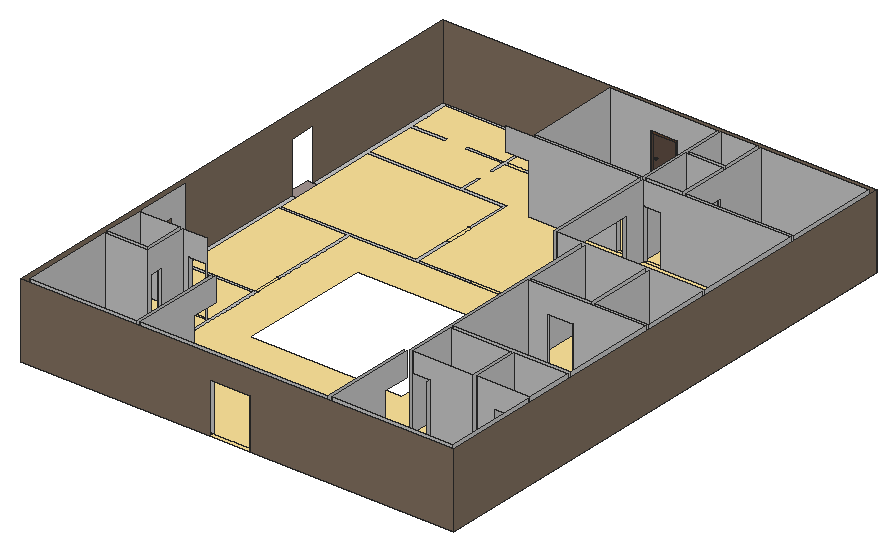
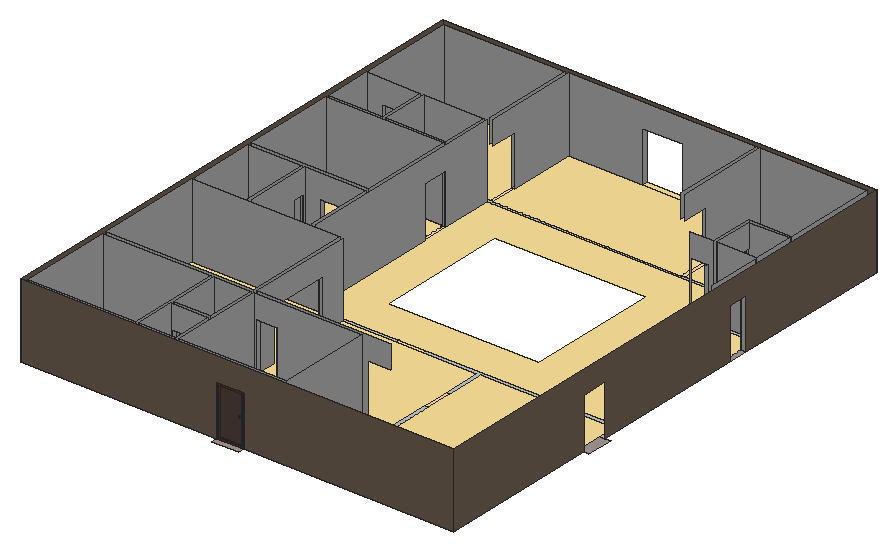
# SketchUp Ruby script. Lengths in inches.
U = 1.inch
M = Sketchup.active_model
def pt(a) = Geom::Point3d.new(a.map { |v| v * U })
def face(e, loops, mat)
  f = e.add_face(loops[0].map { |a| pt(a) })
  loops[1..].each { |l| e.add_face(l.map { |a| pt(a) }).erase! }
  f.material = f.back_material = mat if mat
  f
end
# faces: each face lists its corners as indices into pts; further lists are holes
def faces(e, pts, list, mat = nil) = list.each { |f| face(e, (f[0].is_a?(Array) ? f : [f]).map { |l| l.map { |i| pts[i] } }, mat) }
# xy, xz, yz: faces in a plane at the given z, y or x. An outline is a flat list of corners, or four numbers for a rectangle; further outlines are holes
def ring(l) = l.size == 4 ? [[l[0], l[1]], [l[2], l[1]], [l[2], l[3]], [l[0], l[3]]] : l.each_slice(2).to_a
def flat(e, list, mat, &to3) = list.each { |f| face(e, (f[0].is_a?(Array) ? f : [f]).map { |l| ring(l).map { |u, v| to3.(u, v) } }, mat) }
def xy(e, z, list, mat = nil) = flat(e, list, mat) { |x, y| [x, y, z] }
def xz(e, y, list, mat = nil) = flat(e, list, mat) { |x, z| [x, y, z] }
def yz(e, x, list, mat = nil) = flat(e, list, mat) { |y, z| [x, y, z] }
def lines(e, pts, list) = list.each { |a, b| e.add_line(pt(pts[a]), pt(pts[b])) }
# prism: a flat outline (further loops are holes) pulled along v
def prism(e, loops, v, mat = nil)
  f = face(e, loops, mat); d = Geom::Vector3d.new(v.map { |x| x * U })
  f.pushpull(f.normal.samedirection?(d) ? d.length : -d.length)
end
def box(e, o, s, mat = nil) = prism(e, [[o, [o[0] + s[0], o[1], o[2]], [o[0] + s[0], o[1] + s[1], o[2]], [o[0], o[1] + s[1], o[2]]]], [0, 0, s[2]], mat)
def at(x, y, z, deg = 0) = Geom::Transformation.translation(pt([x, y, z])) * Geom::Transformation.rotation(ORIGIN, Z_AXIS, deg.degrees)
def axes(o, x, y, z) = Geom::Transformation.new([*x, 0, *y, 0, *z, 0, *pt(o).to_a, 1])
def part(name) = M.definitions.add(name)
# library, detail: a bought-in or finely detailed component or shape, given as its bounding box
def library(name, o, s) = part(name).tap { |d| box(d.entities, o, s) }
def detail(e, o, s) = box(e.add_group.entities, o, s)
def put(e, d, t, mat = nil) = e.add_instance(d, t).tap { |i| i.material = mat if mat }
def group(e, t, mat = nil) = e.add_group.tap { |g| g.transformation = t; g.material = mat if mat }.entities
root = M.entities
M.materials.add("Brick_20_1K").color = [126, 109, 93]
M.materials.add("D02_Buttercup_Glow").color = [255, 229, 155]
M.materials.add("M02_Ash_Whisper").color = [196, 196, 196]
M.materials.add("Marble_06_1K").color = [165, 150, 147]
M.materials.add("Metal_06_1K").color = [238, 236, 231]
M.materials.add("Wood_Floor_12_1K").color = [92, 75, 65]
M.materials.add("Wood_Veneer_15_1K").color = [103, 69, 45]
xy(root,36,[[2773.48,806.69,2845.48,815.69],[2443.48,815.69,2635.48,815.69,2635.48,983.69,2563.48,983.69,2563.48,1061.69,2521.48,1061.69,2521.48,983.69,2443.48,983.69],[2641.48,815.69,2977.48,983.69],[2983.48,815.69,3199.48,983.69],[2635.48,935.69,2641.48,983.69],
  [2977.48,935.69,2983.48,983.69],[2773.48,983.69,2845.48,989.69],[2989.48,983.69,3019.48,989.69],[3134.81,983.69,3170.57,989.69],[2443.48,989.69,2515.48,1061.69],
  [2515.48,989.69,2521.48,1013.69],[[2569.48,989.69,2983.48,1373.69],[2641.48,1061.69,2911.48,1301.69]],[2989.48,989.69,3097.48,1073.69],[3103.48,989.69,3199.48,1073.69],[2532.36,1061.69,2562.36,1067.69],
  [2443.48,1067.69,2563.48,1163.69],[2989.48,1079.69,3199.48,1247.69],[2983.48,1081.39,2989.48,1129.39],[2443.48,1169.69,2563.48,1373.69],[2563.48,1169.69,2569.48,1217.69],
  [3021.96,1247.69,3069.96,1253.69],[2989.48,1253.69,3097.48,1373.69],[3103.48,1253.69,3199.48,1373.69],[3097.48,1256.05,3103.48,1280.05],[2785.48,1373.69,2833.48,1379.69],
  [2443.48,1379.69,2683.48,1571.69],[2689.48,1379.69,2929.48,1379.69,2929.48,1425.125,2935.48,1425.125,2935.48,1379.69,3199.48,1379.69,3199.48,1571.69,2935.48,1571.69,2935.48,1534.97,2929.48,1534.97,2929.48,1571.69,2731.48,1571.69,2731.48,1667.69,2611.48,1667.69,2611.48,1641.35,2605.48,1641.35,2605.48,1667.69,2540.32,1667.69,2540.32,1673.69,2605.48,1673.69,2605.48,1745.69,2443.48,1745.69,2443.48,1673.69,2504.32,1673.69,2504.32,1667.69,2443.48,1667.69,2443.48,1577.69,2605.48,1577.69,2605.48,1615.16,2611.48,1615.16,2611.48,1577.69,2689.48,1577.69],[2683.48,1448.15,2689.48,1496.15],[2888.46,1571.69,2924.46,1577.69],[2937.08,1571.69,2967.08,1577.69],
  [2737.48,1577.69,2929.48,1745.69],[2935.48,1577.69,3001.48,1667.69],[3007.48,1577.69,3199.48,1745.69],[3001.48,1619.95,3007.48,1655.95],[2615.5625,1667.69,2645.5625,1673.69],
  [2968.3,1667.69,2998.3,1673.69],[2611.48,1673.69,2731.48,1745.69],[2935.48,1673.69,3001.48,1745.69]],"D02_Buttercup_Glow")
xy(root,36,[[2434.48,806.69,2434.48,1097.3,2443.48,1097.3,2443.48,1067.69,2532.36,1067.69,2532.36,1061.69,2521.48,1061.69,2521.48,1013.69,2515.48,1013.69,2515.48,1061.69,2443.48,1061.69,2443.48,989.69,2521.48,989.69,2521.48,983.69,2443.48,983.69,2443.48,815.69,2635.48,815.69,2635.48,935.69,2641.48,935.69,2641.48,815.69,2773.48,815.69,2773.48,806.69],[2845.48,806.69,2845.48,815.69,2977.48,815.69,2977.48,935.69,2983.48,935.69,2983.48,815.69,3199.48,815.69,3199.48,983.69,3170.57,983.69,3170.57,989.69,3199.48,989.69,3199.48,1073.69,3103.48,1073.69,3103.48,989.69,3134.81,989.69,3134.81,983.69,3019.48,983.69,3019.48,989.69,3097.48,989.69,3097.48,1073.69,2989.48,1073.69,2989.48,983.69,2845.48,983.69,2845.48,989.69,2983.48,989.69,2983.48,1081.39,2989.48,1081.39,2989.48,1079.69,3199.48,1079.69,3199.48,1247.69,3069.96,1247.69,3069.96,1253.69,3097.48,1253.69,3097.48,1256.05,3103.48,1256.05,3103.48,1253.69,3199.48,1253.69,3199.48,1373.69,3103.48,1373.69,3103.48,1280.05,3097.48,1280.05,3097.48,1373.69,2989.48,1373.69,2989.48,1253.69,3021.96,1253.69,3021.96,1247.69,2989.48,1247.69,2989.48,1129.39,2983.48,1129.39,2983.48,1373.69,2833.48,1373.69,2833.48,1379.69,2929.48,1379.69,2929.48,1425.125,2935.48,1425.125,2935.48,1379.69,3199.48,1379.69,3199.48,1571.69,2967.08,1571.69,2967.08,1577.69,3001.48,1577.69,3001.48,1619.95,3007.48,1619.95,3007.48,1577.69,3199.48,1577.69,3199.48,1745.69,3007.48,1745.69,3007.48,1655.95,3001.48,1655.95,3001.48,1667.69,2998.3,1667.69,2998.3,1673.69,3001.48,1673.69,3001.48,1745.69,2935.48,1745.69,2935.48,1673.69,2968.3,1673.69,2968.3,1667.69,2935.48,1667.69,2935.48,1577.69,2937.08,1577.69,2937.08,1571.69,2935.48,1571.69,2935.48,1534.97,2929.48,1534.97,2929.48,1571.69,2924.46,1571.69,2924.46,1577.69,2929.48,1577.69,2929.48,1745.69,2857.48,1745.69,2857.48,1751.69,3208.48,1751.69,3208.48,806.69],[2563.48,983.69,2563.48,1061.69,2562.36,1061.69,2562.36,1067.69,2563.48,1067.69,2563.48,1163.69,2443.48,1163.69,2443.48,1133.3,2434.48,1133.3,2434.48,1412.46,2443.48,1412.46,2443.48,1379.69,2683.48,1379.69,2683.48,1448.15,2689.48,1448.15,2689.48,1379.69,2785.48,1379.69,2785.48,1373.69,2569.48,1373.69,2569.48,1217.69,2563.48,1217.69,2563.48,1373.69,2443.48,1373.69,2443.48,1169.69,2569.48,1169.69,2569.48,989.69,2773.48,989.69,2773.48,983.69],[2434.48,1460.46,2434.48,1751.69,2809.48,1751.69,2809.48,1745.69,2737.48,1745.69,2737.48,1577.69,2888.46,1577.69,2888.46,1571.69,2731.48,1571.69,2731.48,1667.69,2645.5625,1667.69,2645.5625,1673.69,2731.48,1673.69,2731.48,1745.69,2611.48,1745.69,2611.48,1673.69,2615.5625,1673.69,2615.5625,1667.69,2611.48,1667.69,2611.48,1641.35,2605.48,1641.35,2605.48,1667.69,2540.32,1667.69,2540.32,1673.69,2605.48,1673.69,2605.48,1745.69,2443.48,1745.69,2443.48,1673.69,2504.32,1673.69,2504.32,1667.69,2443.48,1667.69,2443.48,1577.69,2605.48,1577.69,2605.48,1615.16,2611.48,1615.16,2611.48,1577.69,2689.48,1577.69,2689.48,1496.15,2683.48,1496.15,2683.48,1571.69,2443.48,1571.69,2443.48,1460.46]],"M02_Ash_Whisper")
xy(root,36,[[2434.48,1097.3,2443.48,1133.3],[2424.79,1412.46,2443.48,1460.46],[2809.48,1745.69,2857.48,1761.69]],"Marble_06_1K")
xz(root,806.69,[[2434.48,36,2773.48,36,2773.48,126,2845.48,126,2845.48,36,3208.48,36,3208.48,168,2434.48,168]],"Brick_20_1K")
xz(root,815.69,[[2443.48,36,2635.48,168],[2641.48,36,2641.48,168,2977.48,168,2977.48,36,2845.48,36,2845.48,126,2773.48,126,2773.48,36],[2983.48,36,3199.48,168]],"M02_Ash_Whisper")
xz(root,983.69,[[2443.48,36,2521.48,168]],"M02_Ash_Whisper")
xz(root,989.69,[[2443.48,36,2515.48,168],[2515.48,36,2521.48,126],[3019.48,36,3019.48,132,2989.48,132,2989.48,168,3097.48,168,3097.48,36],[3103.48,36,3103.48,168,3199.48,168,3199.48,36,3170.57,36,3170.57,126,3134.81,126,3134.81,36]],"M02_Ash_Whisper")
xz(root,1013.69,[[2515.48,36,2521.48,126]],"M02_Ash_Whisper")
xz(root,1061.69,[[2443.48,36,2515.48,168],[2521.48,36,2532.36,36,2532.36,126,2562.36,126,2562.36,36,2563.48,36,2563.48,168,2521.48,168]],"M02_Ash_Whisper")
xz(root,1073.69,[[2989.48,36,3097.48,168],[3103.48,36,3199.48,168]],"M02_Ash_Whisper")
xz(root,1079.69,[[2989.48,36,3199.48,168]],"M02_Ash_Whisper")
xz(root,1097.3,[[2434.48,36,2443.48,126]],"M02_Ash_Whisper")
xz(root,1129.39,[[2983.48,36,2989.48,126]],"M02_Ash_Whisper")
xz(root,1247.69,[[2989.48,36,3021.96,36,3021.96,126,3069.96,126,3069.96,36,3199.48,36,3199.48,168,2989.48,168]],"M02_Ash_Whisper")
xz(root,1253.69,[[2989.48,36,2989.48,168,3097.48,168,3097.48,36,3069.96,36,3069.96,126,3021.96,126,3021.96,36],[3103.48,36,3199.48,168]],"M02_Ash_Whisper")
xz(root,1280.05,[[3097.48,36,3103.48,126]],"M02_Ash_Whisper")
xz(root,1379.69,[[2935.48,36,3199.48,168]],"M02_Ash_Whisper")
xz(root,1425.125,[[2929.48,36,2935.48,126]],"M02_Ash_Whisper")
xz(root,1571.69,[[2731.48,36,2888.46,36,2888.46,126,2924.46,126,2924.46,36,2929.48,36,2929.48,168,2689.48,168,2689.48,126,2731.48,126],[2935.48,36,2937.08,36,2937.08,126,2967.08,126,2967.08,36,3199.48,36,3199.48,168,2935.48,168]],"M02_Ash_Whisper")
xz(root,1577.69,[[2737.48,36,2737.48,168,2929.48,168,2929.48,36,2924.46,36,2924.46,126,2888.46,126,2888.46,36],[2935.48,36,2935.48,168,3001.48,168,3001.48,36,2967.08,36,2967.08,126,2937.08,126,2937.08,36],[3007.48,36,3199.48,168]],"M02_Ash_Whisper")
xz(root,1619.95,[[3001.48,36,3007.48,126]],"M02_Ash_Whisper")
xz(root,1655.95,[[3001.48,36,3007.48,126]],"M02_Ash_Whisper")
xz(root,1667.69,[[2935.48,36,2968.3,36,2968.3,126,2998.3,126,2998.3,36,3001.48,36,3001.48,168,2935.48,168]],"M02_Ash_Whisper")
xz(root,1673.69,[[2935.48,36,2935.48,168,3001.48,168,3001.48,36,2998.3,36,2998.3,126,2968.3,126,2968.3,36]],"M02_Ash_Whisper")
xz(root,1745.69,[[2737.48,36,2809.48,36,2809.48,126,2857.48,126,2857.48,36,2929.48,36,2929.48,168,2737.48,168],[2935.48,36,3001.48,168],[3007.48,36,3199.48,168]],"M02_Ash_Whisper")
xz(root,1751.69,[[2434.48,36,2434.48,168,3208.48,168,3208.48,36,2857.48,36,2857.48,126,2809.48,126,2809.48,36]],"Brick_20_1K")
yz(root,2434.48,[[806.69,36,806.69,168,1751.69,168,1751.69,36,1460.46,36,1460.46,126,1412.46,126,1412.46,36,1133.3,36,1133.3,126,1097.3,126,1097.3,36]],"Brick_20_1K")
yz(root,2443.48,[[815.69,36,983.69,168],[989.69,36,1061.69,168],[1067.69,36,1097.3,36,1097.3,126,1133.3,126,1133.3,36,1163.69,36,1163.69,168,1067.69,168]],"M02_Ash_Whisper")
yz(root,2515.48,[[1013.69,36,1013.69,126,989.69,126,989.69,168,1061.69,168,1061.69,36]],"M02_Ash_Whisper")
yz(root,2521.48,[[983.69,36,989.69,36,989.69,126,1013.69,126,1013.69,36,1061.69,36,1061.69,168,983.69,168]],"M02_Ash_Whisper")
yz(root,2532.36,[[1061.69,36,1067.69,126]],"M02_Ash_Whisper")
yz(root,2635.48,[[815.69,36,815.69,168,983.69,168,983.69,126,935.69,126,935.69,36]],"M02_Ash_Whisper")
yz(root,2641.48,[[815.69,36,935.69,36,935.69,126,983.69,126,983.69,168,815.69,168]],"M02_Ash_Whisper")
yz(root,2737.48,[[1577.69,36,1745.69,168]],"M02_Ash_Whisper")
yz(root,2809.48,[[1745.69,36,1751.69,126]],"M02_Ash_Whisper")
yz(root,2845.48,[[806.69,36,815.69,126]],"M02_Ash_Whisper")
yz(root,2857.48,[[1745.69,36,1751.69,126]],"M02_Ash_Whisper")
yz(root,2888.46,[[1571.69,36,1577.69,126]],"M02_Ash_Whisper")
yz(root,2924.46,[[1571.69,36,1577.69,126]],"M02_Ash_Whisper")
yz(root,2929.48,[[1379.69,36,1379.69,168,1571.69,168,1571.69,36,1534.97,36,1534.97,126,1425.125,126,1425.125,36],[1577.69,36,1745.69,168]],"M02_Ash_Whisper")
yz(root,2935.48,[[1379.69,36,1425.125,36,1425.125,126,1534.97,126,1534.97,36,1571.69,36,1571.69,168,1379.69,168],[1577.69,36,1667.69,168],[1673.69,36,1745.69,168]],"M02_Ash_Whisper")
yz(root,2937.08,[[1571.69,36,1577.69,126]],"M02_Ash_Whisper")
yz(root,2968.3,[[1667.69,36,1673.69,126]],"M02_Ash_Whisper")
yz(root,2977.48,[[815.69,36,815.69,168,983.69,168,983.69,126,935.69,126,935.69,36]],"M02_Ash_Whisper")
yz(root,2983.48,[[815.69,36,935.69,36,935.69,126,983.69,126,983.69,168,815.69,168],[989.69,36,989.69,168,1373.69,168,1373.69,36,1129.39,36,1129.39,126,1081.39,126,1081.39,36]],"M02_Ash_Whisper")
yz(root,2989.48,[[989.69,36,1073.69,168],[1079.69,36,1081.39,36,1081.39,126,1129.39,126,1129.39,36,1247.69,36,1247.69,168,1079.69,168],[1253.69,36,1373.69,168]],"M02_Ash_Whisper")
yz(root,2998.3,[[1667.69,36,1673.69,126]],"M02_Ash_Whisper")
yz(root,3001.48,[[1577.69,36,1577.69,168,1667.69,168,1667.69,36,1655.95,36,1655.95,126,1619.95,126,1619.95,36],[1673.69,36,1745.69,168]],"M02_Ash_Whisper")
yz(root,3007.48,[[1577.69,36,1619.95,36,1619.95,126,1655.95,126,1655.95,36,1745.69,36,1745.69,168,1577.69,168]],"M02_Ash_Whisper")
yz(root,3019.48,[[983.69,36,989.69,132]],"M02_Ash_Whisper")
yz(root,3069.96,[[1247.69,36,1253.69,126]],"M02_Ash_Whisper")
yz(root,3097.48,[[989.69,36,1073.69,168],[1253.69,36,1253.69,168,1373.69,168,1373.69,36,1280.05,36,1280.05,126,1256.05,126,1256.05,36]],"M02_Ash_Whisper")
yz(root,3103.48,[[989.69,36,1073.69,168],[1253.69,36,1256.05,36,1256.05,126,1280.05,126,1280.05,36,1373.69,36,1373.69,168,1253.69,168]],"M02_Ash_Whisper")
yz(root,3170.57,[[983.69,36,989.69,126]],"M02_Ash_Whisper")
yz(root,3199.48,[[815.69,36,983.69,168],[989.69,36,1073.69,168],[1079.69,36,1247.69,168],[1253.69,36,1373.69,168],[1379.69,36,1571.69,168],
  [1577.69,36,1745.69,168]],"M02_Ash_Whisper")
yz(root,3208.48,[[806.69,36,1751.69,168]],"Brick_20_1K")
p = [[2761.29,686.54,36],[2754.29,686.54,36]]
lines(root,p,[[0,1]])
g1 = group(root,at(2809.48,1745.69,36))
xy(g1,0,[[0,0,48,6]],"Wood_Veneer_15_1K")
xy(g1,3,[[3,0,45,2]],"Wood_Floor_12_1K")
xy(g1,3,[[3,2,45,6]],"Wood_Veneer_15_1K")
xy(g1,87,[[3,0,45,2]],"Wood_Floor_12_1K")
xy(g1,87,[[3,2,45,6]],"Wood_Veneer_15_1K")
xy(g1,90,[[0,0,48,6]],"Wood_Veneer_15_1K")
xz(g1,0,[[[0,0,48,90],[3,3,45,87]]],"Wood_Veneer_15_1K")
xz(g1,2,[[3,3,45,87]],"Wood_Floor_12_1K")
xz(g1,6,[[[0,0,48,90],[3,3,45,87]]],"Wood_Veneer_15_1K")
yz(g1,0,[[0,0,6,90]],"Wood_Veneer_15_1K")
yz(g1,3,[[0,3,2,87]],"Wood_Floor_12_1K")
yz(g1,3,[[2,3,6,87]],"Wood_Veneer_15_1K")
yz(g1,45,[[0,3,2,87]],"Wood_Floor_12_1K")
yz(g1,45,[[2,3,6,87]],"Wood_Veneer_15_1K")
yz(g1,48,[[0,0,6,90]],"Wood_Veneer_15_1K")
g2 = group(g1,at(11,2,45.16))
prism(g2,[[[-3.93,0,1.48],[-3.73,0,1],[-3.41,0,0.59],[-3,0,0.27],[-2.52,0,0.07],[-2,0,0],[-1.48,0,0.07],[-1,0,0.27],[-0.59,0,0.59],[-0.27,0,1],[-0.07,0,1.48],[0,0,2],[-0.07,0,2.52],[-0.27,0,3],[-0.59,0,3.41],[-1,0,3.73],[-1.48,0,3.93],[-2,0,4],[-2.52,0,3.93],[-3,0,3.73],[-3.41,0,3.41],[-3.73,0,3],[-3.93,0,2.52],[-4,0,2]]],[0,0.6875,0],"Metal_06_1K")
